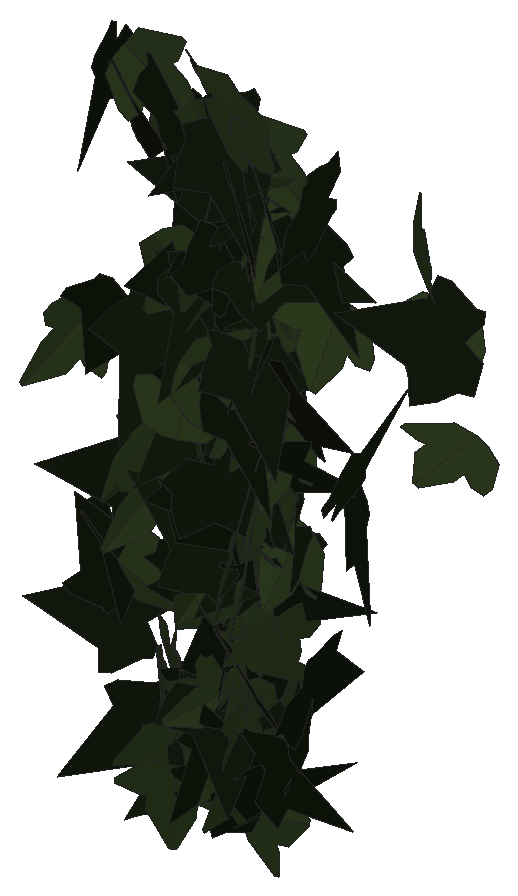
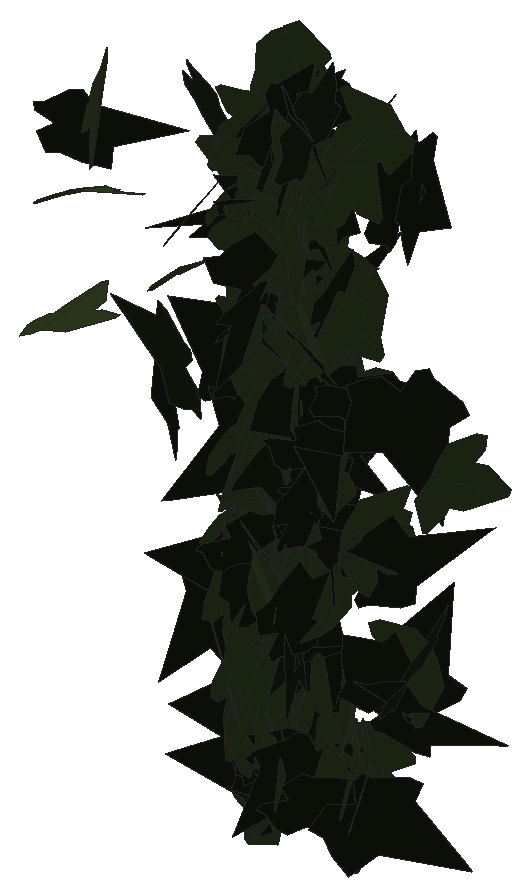
# SketchUp Ruby script. Lengths in inches.
U = 1.inch
M = Sketchup.active_model
def pt(a) = Geom::Point3d.new(a.map { |v| v * U })
def face(e, loops, mat)
  f = e.add_face(loops[0].map { |a| pt(a) })
  loops[1..].each { |l| e.add_face(l.map { |a| pt(a) }).erase! }
  f.material = f.back_material = mat if mat
  f
end
# faces: each face lists its corners as indices into pts; further lists are holes
def faces(e, pts, list, mat = nil) = list.each { |f| face(e, (f[0].is_a?(Array) ? f : [f]).map { |l| l.map { |i| pts[i] } }, mat) }
# xy, xz, yz: faces in a plane at the given z, y or x. An outline is a flat list of corners, or four numbers for a rectangle; further outlines are holes
def ring(l) = l.size == 4 ? [[l[0], l[1]], [l[2], l[1]], [l[2], l[3]], [l[0], l[3]]] : l.each_slice(2).to_a
def flat(e, list, mat, &to3) = list.each { |f| face(e, (f[0].is_a?(Array) ? f : [f]).map { |l| ring(l).map { |u, v| to3.(u, v) } }, mat) }
def xy(e, z, list, mat = nil) = flat(e, list, mat) { |x, y| [x, y, z] }
def xz(e, y, list, mat = nil) = flat(e, list, mat) { |x, z| [x, y, z] }
def yz(e, x, list, mat = nil) = flat(e, list, mat) { |y, z| [x, y, z] }
def lines(e, pts, list) = list.each { |a, b| e.add_line(pt(pts[a]), pt(pts[b])) }
# prism: a flat outline (further loops are holes) pulled along v
def prism(e, loops, v, mat = nil)
  f = face(e, loops, mat); d = Geom::Vector3d.new(v.map { |x| x * U })
  f.pushpull(f.normal.samedirection?(d) ? d.length : -d.length)
end
def box(e, o, s, mat = nil) = prism(e, [[o, [o[0] + s[0], o[1], o[2]], [o[0] + s[0], o[1] + s[1], o[2]], [o[0], o[1] + s[1], o[2]]]], [0, 0, s[2]], mat)
def at(x, y, z, deg = 0) = Geom::Transformation.translation(pt([x, y, z])) * Geom::Transformation.rotation(ORIGIN, Z_AXIS, deg.degrees)
def axes(o, x, y, z) = Geom::Transformation.new([*x, 0, *y, 0, *z, 0, *pt(o).to_a, 1])
def part(name) = M.definitions.add(name)
# library, detail: a bought-in or finely detailed component or shape, given as its bounding box
def library(name, o, s) = part(name).tap { |d| box(d.entities, o, s) }
def detail(e, o, s) = box(e.add_group.entities, o, s)
def put(e, d, t, mat = nil) = e.add_instance(d, t).tap { |i| i.material = mat if mat }
def group(e, t, mat = nil) = e.add_group.tap { |g| g.transformation = t; g.material = mat if mat }.entities
root = M.entities
M.materials.add("efeu1").color = [18, 25, 13]
M.materials.add("efeu2").color = [43, 57, 29]
c1 = part("ivyleaf_9")
p = [[1.54,2.16,1.25],[1.36,2.04,1.19],[-0.21,0.99,0.68],[-0.71,1.11,0.82],[-0.85,0.86,0.67],[-0.8,0.17,0.21],
  [-0.9,-0.01,0.1],[-0.67,-0.16,-0.02],[-0.08,-0.08,-0.05],[-0.03,-0.6,-0.4],[0.65,-0.88,-0.66],[0.83,-0.6,-0.49],
  [1.29,-0.42,-0.43],[1.8125,-0.07,-0.26],[1.21,0.44,0.15]]
faces(c1.entities,p,[[0,1,2,3,4,5,6,7,8,9,10,11,12,13,14]],"efeu1")
c2 = part("ivyleaf_10")
p = [[0,0.5,-0.03],[-0.0625,2.02,-0.43],[-0.19,2.01,-0.46],[-0.54,1.05,-0.29],[-0.52,0.625,-0.18],[-0.83,0.76,-0.28],
  [-1.16,0.64,-0.33],[-1.15,0.33,-0.24],[-0.77,-0.39,0.02],[-0.3,-0.51,0.16],[0.04,-0.48,0.23],[-0.02,2.01,-0.4375],
  [-0.06,2.01,-0.43],[0.04,-0.49,0.23],[0.67,-0.49,0.14],[1.38,0.36,-0.2],[1.375,0.51,-0.24],[0.81,0.65,-0.19],
  [0.62,0.59,-0.15],[0.6,1.09,-0.28],[0.5,1.23,-0.31]]
faces(c2.entities,p,[[0,1,2,3,4,5,6,7,8,9,10],[11,12,0,13,14,15,16,17,18,19,20]],"efeu2")
put(root,c1,axes([47.32,221.0625,219.91],[0.04753,-0.49581,-0.04378],[0.04891,0.04842,-0.49524],[0.49533,0.0428,0.0531]))
put(root,c1,axes([47.02,221.03,219.27],[0.22568,-0.44566,0.02142],[0.01272,-0.01757,-0.49953],[0.44599,0.22601,0.00341]))
put(root,c1,axes([50.25,221.08,221.11],[-0.22275,-0.24833,-0.37244],[-0.25181,-0.27444,0.33358],[-0.3701,0.33618,-0.0028]))
put(root,c1,axes([46.89,221.18,220.5],[-0.38371,-0.31961,0.02478],[-0.01873,-0.01624,-0.49939],[0.32002,-0.38417,0.00049]))
put(root,c1,axes([48.73,221.12,218.4375],[-0.08228,-0.03825,-0.4917],[0.49018,-0.06123,-0.07726],[-0.05431,-0.49476,0.04758]))
put(root,c1,axes([47.24,220.95,221.98],[-0.26948,0.0763,0.4142],[-0.39639,0.12021,-0.28004],[-0.14232,-0.4793,-0.0043]))
put(root,c2,axes([46.32,220.93,214.18],[-0.43141,-0.24475,0.0631],[-0.05478,-0.03132,-0.496],[0.24675,-0.43487,0.0002]))
put(root,c2,axes([47.07,221.22,215.55],[0.11367,0.11828,-0.47232],[-0.30961,-0.35678,-0.16386],[-0.3758,0.32972,-0.00787]))
put(root,c1,axes([46.95,221.09,215.5],[-0.20811,-0.41168,-0.19289],[0.07628,0.17752,-0.46116],[0.44819,-0.22137,-0.01108]))
put(root,c2,axes([46.91,220.63,219.75],[0.12856,0.23562,0.42185],[0.11779,0.40807,-0.26383],[-0.46861,0.16721,0.04941]))
put(root,c1,axes([46.99,221.07,222.54],[0.00321,-0.47356,-0.16042],[0.00882,0.16045,-0.47348],[0.49991,0.00021,0.00938]))
put(root,c2,axes([46.46,220.84,218.9375],[0.40963,0.27351,-0.08599],[0.06979,0.05032,0.49254],[0.27809,-0.41552,0.00305]))
put(root,c2,axes([46.96,221.06,215.37],[-0.4493,-0.21591,-0.03894],[-0.03223,-0.02283,0.49844],[-0.21701,0.4504,0.0066]))
put(root,c1,axes([46.95,221.23,221.85],[0.16787,-0.04444,-0.46887],[0.44681,-0.14237,0.17347],[-0.14892,-0.47724,-0.00808]))
put(root,c2,axes([47.16,220.92,222.83],[-0.4681,0.01568,0.17503],[-0.17518,-0.00218,-0.4683],[-0.01393,-0.49975,0.00753]))
put(root,c2,axes([47.25,221.08,218.35],[0.31151,-0.39083,0.0145],[0.00934,-0.01109,-0.49979],[0.39099,0.31165,0.00039]))
put(root,c1,axes([46.83,221.13,215.36],[0.43801,0.0262,0.23972],[-0.24022,0.00396,0.43849],[0.02107,-0.4993,0.01606]))
put(root,c2,axes([46.16,221.02,214.71],[-0.183,-0.46294,-0.04694],[0.01727,0.04364,-0.49779],[0.46499,-0.18381,0.00002]))
put(root,c1,axes([46.92,221.08,217.3125],[-0.37101,-0.22666,-0.24693],[-0.21231,-0.12612,0.43476],[-0.25937,0.42746,-0.00266]))
put(root,c1,axes([48.32,221.09,222.24],[-0.4251,0.23085,-0.12646],[0.10723,-0.0675,-0.48368],[-0.24039,-0.43835,0.00788]))
put(root,c1,axes([46.9375,221.13,216.94],[0.2473,-0.04784,0.43192],[-0.41996,0.10143,0.25169],[-0.1117,-0.48726,0.00999]))
put(root,c2,axes([47.09,221.27,215.2],[0.17477,-0.39638,0.24967],[0.10141,-0.22815,-0.4332],[0.45735,0.20206,0.00065]))
put(root,c2,axes([47.16,220.99,223.07],[-0.40341,0.00961,0.29524],[-0.29525,-0.02855,-0.40251],[0.00912,-0.49909,0.02871]))
put(root,c2,axes([47.26,221.3,219.01],[-0.2017,-0.18431,-0.41874],[-0.32399,-0.26557,0.27295],[-0.32303,0.38145,-0.0123]))
put(root,c2,axes([47.04,221.41,216.7],[-0.05338,-0.05157,0.49446],[-0.04641,-0.49461,-0.0566],[0.49497,-0.05194,0.04802]))
put(root,c1,axes([46.94,220.875,218.41],[-0.04688,-0.2042,-0.45399],[0.07241,0.44835,-0.20914],[0.4925,-0.08535,-0.01246]))
put(root,c1,axes([47.02,220.77,220.85],[-0.04978,-0.03478,0.4963],[0.41951,0.26519,0.06067],[-0.26745,0.42245,0.00278]))
put(root,c1,axes([46.98,221.44,222.55],[0.00255,-0.13751,-0.48071],[0.10544,-0.46976,0.13494],[-0.48875,-0.10206,0.0266]))
put(root,c1,axes([46.92,220.77,221.26],[0.03686,0.1182,-0.48443],[0.18371,0.44836,0.12338],[0.46356,-0.18709,-0.01038]))
put(root,c1,axes([46.83,221,220.54],[-0.24684,0.28167,0.33126],[0.20737,-0.25855,0.37437],[0.38219,0.3222,0.01082]))
put(root,c2,axes([47.08,221.38,217.3],[-0.01866,-0.00486,-0.49963],[0.23493,-0.44135,-0.00448],[-0.44098,-0.23492,0.01876]))
put(root,c1,axes([47.375,221.05,214.74],[0.1383,0.04143,-0.4787],[0.42811,0.21554,0.14234],[0.21816,-0.44925,0.02414]))
put(root,c1,axes([47.04,221.22,214.95],[-0.00935,0.26908,-0.42132],[-0.00487,-0.42142,-0.26904],[-0.49989,-0.00093,0.01051]))
put(root,c2,axes([47.49,221.45,221.39],[-0.30162,-0.21874,0.33343],[0.21417,-0.44151,-0.09591],[0.33639,0.08496,0.36003]))
put(root,c2,axes([46.6,220.98,214.49],[0.03985,-0.00403,-0.49839],[-0.44376,0.22735,-0.03732],[0.22692,0.44531,0.01454]))
put(root,c1,axes([47.26,221.43,221.56],[0.03941,-0.16409,0.47066],[0.12986,-0.45245,-0.16861],[0.48123,0.13553,0.00695]))
put(root,c1,axes([46.92,221.26,214.18],[0.39148,0.05181,0.3067],[-0.30399,-0.04067,0.39489],[0.06586,-0.49564,-0.00034]))
put(root,c2,axes([47.07,221.32,217.54],[0.31767,-0.29695,0.24679],[0.17649,-0.17257,-0.43482],[0.34342,0.36337,-0.00482]))
put(root,c1,axes([47.2,221.27,215.46],[0.2348,-0.3957,0.19567],[-0.10344,0.16614,0.46011],[-0.42915,-0.25655,-0.00384]))
put(root,c2,axes([46.875,221.07,215.45],[-0.47578,0.14898,0.03797],[-0.03837,0.00452,-0.49851],[-0.14887,-0.47727,0.00713]))
put(root,c2,axes([46.15,221.04,215.74],[-0.38222,0.30622,0.1007],[-0.07846,0.06313,-0.48975],[-0.31266,-0.39019,-0.00021]))
put(root,c2,axes([47.51,221.55,217.36],[-0.30196,-0.20582,0.34126],[0.21426,-0.44486,-0.07871],[0.33603,0.0987,0.35685]))
put(root,c2,axes([46.76,221.13,219.08],[-0.44376,0.21366,-0.08617],[0.0812,-0.02997,-0.49245],[-0.2156,-0.45105,-0.0081]))
put(root,c1,axes([46.16,221.58,220.35],[-0.09147,-0.12517,0.47536],[-0.18531,-0.43906,-0.15127],[0.45529,-0.20386,0.03393]))
put(root,c2,axes([46.72,220.91,221.0625],[-0.07109,-0.27638,-0.41056],[0.13852,0.38709,-0.28456],[0.47514,-0.1542,0.02153]))
put(root,c1,axes([47.5625,221.37,219.25],[0.19213,-0.18313,0.42373],[0.28896,-0.31021,-0.26509],[0.35998,0.34675,-0.01336]))
put(root,c2,axes([46.59,221.13,216.35],[-0.06684,-0.46393,0.17406],[0.02403,0.1724,0.46872],[-0.49493,0.07102,-0.00075]))
put(root,c2,axes([47.16,221.12,217.32],[-0.46371,0.04013,0.18264],[-0.18139,0.02222,-0.46541],[-0.04547,-0.49789,-0.00605]))
put(root,c1,axes([48.64,220.97,218.6],[-0.18633,0.4616,0.04699],[0.01116,-0.04617,0.49774],[0.46385,0.18654,0.00691]))
put(root,c2,axes([45.68,221.47,217.5625],[0.14778,0.29132,-0.37854],[-0.18849,-0.32852,-0.32641],[-0.4389,0.23918,0.01273]))
put(root,c2,axes([47.15,221.09,214.41],[-0.08734,-0.42131,-0.2547],[0.06395,0.24677,-0.43013],[0.48814,-0.10771,0.01078]))
put(root,c2,axes([46.99,221.33,220.16],[0.39896,-0.30133,-0.00534],[-0.00451,0.0029,-0.49997],[0.30135,0.39899,-0.00041]))
put(root,c2,axes([46.81,221.23,216.78],[-0.46773,0.00753,-0.17657],[0.17577,-0.03204,-0.46699],[-0.01835,-0.49892,0.02733]))
put(root,c2,axes([45.98,221.25,220.7],[-0.38148,0.0254,-0.32222],[0.31742,-0.0646,-0.38088],[-0.06098,-0.49516,0.03316]))
put(root,c2,axes([47.24,221.57,215.93],[0.01182,-0.36876,0.33746],[0.00465,-0.33745,-0.36892],[0.49984,0.01186,-0.00455]))
put(root,c1,axes([46.67,221.4375,222.5625],[-0.29551,-0.01886,-0.40289],[0.40333,-0.01155,-0.29529],[0.00183,-0.49951,0.02204]))
put(root,c1,axes([46.53,221.68,217.72],[-0.08612,-0.14445,0.47087],[-0.24272,-0.40349,-0.16817],[0.42857,-0.25755,-0.00063]))
put(root,c2,axes([47.54,221.25,216.41],[-0.17608,-0.4598,-0.08706],[0.03297,0.0806,-0.49236],[0.46681,-0.17913,0.00193]))
put(root,c1,axes([45.82,221.6,222.48],[0.0679,-0.44691,0.21369],[0.04612,-0.20905,-0.45185],[0.49322,0.08107,0.01283]))
put(root,c1,axes([47.16,220.98,219.45],[-0.36383,0.26895,-0.21283],[-0.17959,0.11495,0.45225],[0.29219,0.40553,0.01296]))
put(root,c2,axes([48,221.67,220.33],[-0.3874,-0.23225,0.21443],[0.21959,-0.44171,-0.08169],[0.22738,0.03087,0.44424]))
put(root,c1,axes([45.75,221.55,219.54],[-0.35499,-0.34787,-0.05444],[0.03749,0.03953,-0.49702],[0.35011,-0.35696,-0.00199]))
put(root,c1,axes([47.1,220.97,214.12],[0.08474,0.37598,-0.31853],[0.06154,0.3126,0.38535],[0.48891,-0.10452,0.0067]))
put(root,c2,axes([47.1,221.46,213.8],[0.10193,-0.11272,-0.47635],[0.41099,-0.24459,0.14582],[-0.26589,-0.42127,0.04279]))
put(root,c2,axes([46.71,221.29,220.34],[-0.01132,-0.48832,-0.10683],[-0.00772,0.10702,-0.48835],[0.49981,-0.00941,-0.00997]))
put(root,c2,axes([46.72,221.07,221.88],[0.1182,-0.26065,-0.40999],[-0.11432,0.39518,-0.28419],[0.47219,0.16093,0.03382]))
put(root,c1,axes([47.04,221.54,214.47],[-0.1383,-0.18521,-0.44336],[-0.2769,-0.34633,0.23105],[-0.39268,0.30944,-0.00677]))
put(root,c1,axes([45.14,221.58,222.02],[0.08367,-0.16478,0.46459],[0.23355,-0.40174,-0.18455],[0.43411,0.2479,0.00974]))
put(root,c2,axes([46.98,221.33,217.29],[-0.3686,-0.19313,0.2772],[0.2564,0.10723,0.41565],[-0.21999,0.44856,0.01999]))
put(root,c2,axes([47.08,221.1,221.41],[0.07492,-0.09155,-0.4858],[-0.30509,0.37805,-0.11829],[0.38898,0.31415,0.00078]))
put(root,c1,axes([47.25,221.17,221.15],[0.31354,-0.24842,-0.29997],[0.15983,0.43324,-0.19172],[0.35517,0.02433,0.35109]))
put(root,c1,axes([48.14,220.96,215.98],[-0.06849,0.09938,-0.48521],[-0.29654,0.38411,0.12053],[0.3967,0.30428,0.00632]))
put(root,c2,axes([47.16,221.66,215.04],[0.01283,-0.37068,0.33531],[0.02533,-0.33451,-0.37076],[0.49919,0.0265,0.0102]))
put(root,c2,axes([47.02,221.24,218.99],[-0.39811,0.20296,0.22432],[-0.21736,0.06596,-0.44543],[-0.2104,-0.45217,0.03571]))
put(root,c1,axes([47.13,221.26,216.68],[0.29404,-0.02715,0.40349],[0.40379,-0.00778,-0.29478],[0.02229,0.4992,0.01735]))
put(root,c2,axes([46.92,221.15,217.13],[0.10472,-0.30859,-0.37922],[-0.04351,0.3804,-0.32157],[0.48697,0.10035,0.05282]))
put(root,c1,axes([46.61,221.76,216.37],[-0.0706,-0.08727,0.48724],[-0.31408,-0.3725,-0.11223],[0.38258,-0.32191,-0.00223]))
put(root,c2,axes([47.04,221.52,216.59],[0.29687,-0.32009,-0.24374],[0.17903,-0.16616,0.43628],[-0.3603,-0.34631,0.01596]))
put(root,c2,axes([47,221.36,220.25],[0.1647,-0.04989,-0.46945],[-0.4504,0.13238,-0.17209],[0.14146,0.47957,-0.00133]))
put(root,c1,axes([45.4,221.72,217.42],[-0.13565,-0.0828,0.47407],[-0.41474,-0.22973,-0.15879],[0.24411,-0.43631,-0.00636]))
put(root,c1,axes([47.88,221.09,214.92],[0.00226,0.0991,0.49008],[-0.11636,0.47673,-0.09587],[-0.48627,-0.11362,0.02522]))
put(root,c1,axes([47.75,221.49,221.4],[0.23785,-0.43214,-0.08174],[-0.01467,0.08508,-0.49249],[0.43956,0.23668,0.02779]))
put(root,c2,axes([47.21,221.76,218.58],[-0.26221,-0.29591,0.30608],[0.22173,-0.40179,-0.1985],[0.36343,0.03163,0.34193]))
put(root,c2,axes([46.32,221.58,220.01],[0.26044,-0.33343,-0.26645],[0.16502,-0.20921,0.42309],[-0.39362,-0.30832,0.00107]))
put(root,c2,axes([49.46,221.78,220.82],[-0.45096,-0.18857,0.10525],[0.16921,-0.45996,-0.09904],[0.13417,-0.0537,0.47866]))
put(root,c1,axes([45.61,221.66,214.44],[0.00336,0.01525,-0.49976],[-0.18336,-0.46491,-0.01541],[-0.46515,0.18338,0.00247]))
put(root,c2,axes([46.64,221.66,220.03],[0.17054,0.27514,-0.38107],[-0.23058,-0.30427,-0.32288],[-0.40957,0.28586,0.0231]))
put(root,c2,axes([46.21,221.45,218.19],[-0.40574,0.29189,0.01318],[0.00855,-0.01067,0.49981],[0.29206,0.40582,0.00367]))
put(root,c1,axes([44.8,221.77,216.43],[0.09289,-0.37646,0.31567],[0.08133,-0.30505,-0.38772],[0.48452,0.12338,0.00456]))
put(root,c2,axes([47.01,221.31,221.57],[-0.14169,-0.2568,0.40494],[0.3174,0.26628,0.27992],[-0.35942,0.33638,0.08756]))
put(root,c1,axes([46.38,221.36,219.28],[0.21755,0.36712,-0.26057],[-0.12935,-0.22622,-0.42672],[-0.43121,0.25308,-0.00345]))
put(root,c1,axes([46.25,221.72,222.56],[0.15572,-0.29738,0.37057],[0.19396,-0.3162,-0.33525],[0.43374,0.24816,0.01688]))
put(root,c2,axes([44.36,221.74,219.03],[0.11701,0.24376,-0.42058],[-0.19209,-0.3742,-0.27032],[-0.44655,0.22484,0.00608]))
put(root,c1,axes([45.17,221.57,215.96],[0.26882,0.09518,0.4107],[-0.41597,-0.01938,0.27676],[0.0686,-0.49047,0.06877]))
put(root,c1,axes([45.35,221.53,215.63],[-0.3031,0.08903,0.38756],[-0.38502,0.05614,-0.31401],[-0.09943,-0.4888,0.03453]))
put(root,c1,axes([46.92,221.16,216.11],[-0.07063,0.05904,-0.49145],[-0.43979,0.22032,0.08968],[0.22714,0.44494,0.02081]))
put(root,c2,axes([46.97,221.42,219.23],[-0.45708,0.1912,-0.06722],[0.0591,-0.03289,-0.4954],[-0.19387,-0.46082,0.00747]))
put(root,c1,axes([46.98,221.39,220.26],[0.08587,-0.35575,-0.34069],[-0.05945,0.33581,-0.36564],[0.48897,0.1033,0.01538]))
put(root,c2,axes([47.36,221.43,217.97],[0.04761,-0.48434,-0.11468],[0.15493,0.1239,-0.45896],[0.473,0.00816,0.16188]))
put(root,c2,axes([44.98,221.47,216.38],[-0.23249,0.0101,-0.44254],[0.43653,-0.07767,-0.2311],[-0.07341,-0.49383,0.0273]))
put(root,c2,axes([45.54,221.67,214.96],[-0.14732,0.29521,-0.3757],[0.15941,-0.34026,-0.32987],[-0.45043,-0.21697,0.00614]))
put(root,c2,axes([45.66,221.74,215.09],[-0.11225,0.23423,-0.42724],[0.13576,-0.40604,-0.25827],[-0.46794,-0.17399,0.02756]))
put(root,c1,axes([47.23,221.81,217.3],[-0.34244,-0.31647,0.1805],[-0.13214,-0.12296,-0.46628],[0.33952,-0.36705,0.00058]))
put(root,c1,axes([47.15,221.16,218.35],[0.36449,0.23577,0.24811],[0.2086,0.13434,-0.4341],[-0.27136,0.41996,-0.00043]))
put(root,c2,axes([45.42,221.81,217.97],[-0.02304,-0.30545,0.39518],[-0.01747,-0.39487,-0.30622],[0.49916,-0.02792,0.00753]))
put(root,c2,axes([47.0625,221.4,222.32],[0.30542,0.12378,0.37603],[0.33719,0.1675,-0.32901],[-0.20742,0.45456,0.01884]))
put(root,c2,axes([45.38,221.42,222.83],[0.25904,0.10377,0.41488],[0.38604,0.15199,-0.27905],[-0.18403,0.4649,-0.00137]))
put(root,c1,axes([46.35,221.75,218.78],[-0.44038,-0.22705,0.06718],[-0.06098,-0.02832,-0.49546],[0.2288,-0.44457,-0.00274]))
put(root,c1,axes([46.41,221.8,214.3],[-0.39044,-0.24571,0.19284],[-0.16543,-0.09917,-0.4613],[0.26494,-0.42402,-0.00386]))
put(root,c1,axes([47.19,221.66,220.375],[-0.15363,0.01086,0.47569],[-0.47533,-0.02596,-0.15292],[0.02137,-0.49921,0.0183]))
put(root,c2,axes([46.99,221.45,219.78],[0.33693,0.15479,0.33544],[0.31374,0.11981,-0.37042],[-0.19505,0.46009,-0.01639]))
put(root,c2,axes([47.36,221.39,215.45],[-0.11385,-0.44299,-0.20198],[0.05027,0.19562,-0.45739],[0.48426,-0.12446,0]))
put(root,c1,axes([47.44,221.62,217.48],[-0.46929,0.11558,-0.12811],[0.12499,-0.02819,-0.4833],[-0.11895,-0.48564,-0.00243]))
put(root,c2,axes([49.58,221.24,221.94],[-0.22011,0.17511,0.41339],[-0.30705,0.27716,-0.28089],[-0.32753,-0.37751,-0.01448]))
put(root,c1,axes([46.7,221.59,219.9375],[-0.48093,0.13539,0.01935],[-0.01764,0.00876,-0.49961],[-0.13562,-0.48124,-0.00365]))
put(root,c2,axes([49.66,221.9,219.17],[-0.46664,-0.02976,0.1771],[0.07863,-0.47717,0.127],[0.16146,0.14638,0.45]))
put(root,c2,axes([46.01,221.47,222.21],[-0.47096,-0.03891,-0.16334],[0.16301,0.01066,-0.47256],[0.04026,-0.49837,0.00264]))
put(root,c2,axes([46.9375,221.21,214.54],[-0.07357,0.09048,0.48621],[-0.32149,0.36478,-0.11653],[-0.37581,-0.32977,0.0045]))
put(root,c2,axes([46.97,221.4,215.5],[-0.026,-0.43778,-0.24016],[0.03365,0.2384,-0.43822],[0.49819,-0.03895,0.01707]))
put(root,c2,axes([47.11,221.42,218.95],[0.04682,-0.45414,-0.20389],[0.15273,0.20801,-0.42826],[0.4738,-0.02218,0.1582]))
put(root,c1,axes([44.74,221.8,222.64],[-0.12022,0.10392,-0.47408],[0.3765,-0.28824,-0.15865],[-0.30627,-0.39512,-0.00895]))
put(root,c1,axes([45.13,221.52,219.67],[0.19463,0.26851,-0.37419],[-0.23358,-0.29256,-0.33143],[-0.39694,0.30382,0.01156]))
put(root,c1,axes([46.43,221.4375,214.72],[0.02573,-0.28541,-0.40973],[0.07606,0.40773,-0.27924],[0.49351,-0.04795,0.0644]))
put(root,c2,axes([46.875,221.52,221.11],[-0.40313,0.06202,-0.28921],[0.28613,-0.04208,-0.40787],[-0.07493,-0.49435,-0.00156]))
put(root,c2,axes([47.1,221.58,220.91],[-0.46502,0.05221,-0.17615],[0.16013,-0.11983,-0.45825],[-0.09007,-0.48261,0.09473]))
put(root,c2,axes([46.07,221.5,220.37],[-0.33082,-0.29285,-0.2341],[0.24612,0.06588,-0.43022],[0.28282,-0.39988,0.10056]))
